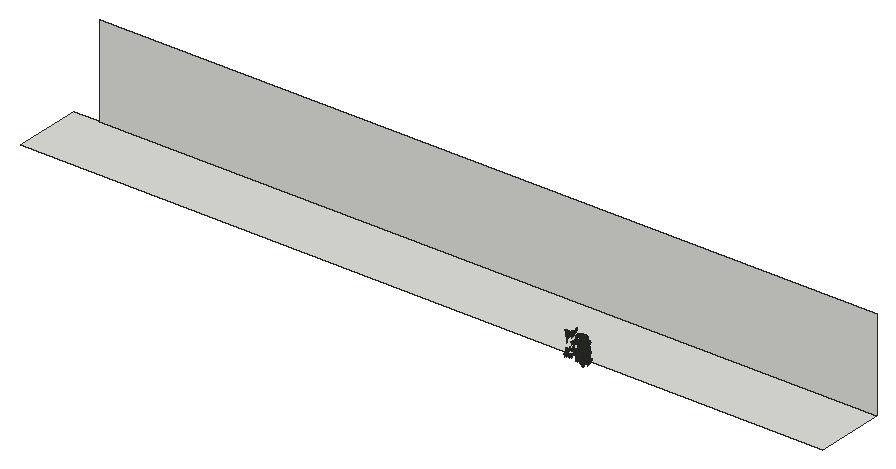
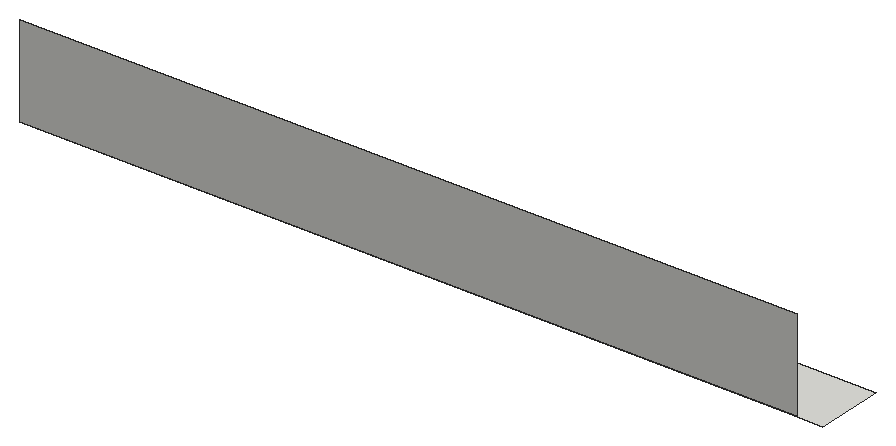
# SketchUp Ruby script. Lengths in inches.
U = 1.inch
M = Sketchup.active_model
def pt(a) = Geom::Point3d.new(a.map { |v| v * U })
def face(e, loops, mat)
  f = e.add_face(loops[0].map { |a| pt(a) })
  loops[1..].each { |l| e.add_face(l.map { |a| pt(a) }).erase! }
  f.material = f.back_material = mat if mat
  f
end
# faces: each face lists its corners as indices into pts; further lists are holes
def faces(e, pts, list, mat = nil) = list.each { |f| face(e, (f[0].is_a?(Array) ? f : [f]).map { |l| l.map { |i| pts[i] } }, mat) }
# xy, xz, yz: faces in a plane at the given z, y or x. An outline is a flat list of corners, or four numbers for a rectangle; further outlines are holes
def ring(l) = l.size == 4 ? [[l[0], l[1]], [l[2], l[1]], [l[2], l[3]], [l[0], l[3]]] : l.each_slice(2).to_a
def flat(e, list, mat, &to3) = list.each { |f| face(e, (f[0].is_a?(Array) ? f : [f]).map { |l| ring(l).map { |u, v| to3.(u, v) } }, mat) }
def xy(e, z, list, mat = nil) = flat(e, list, mat) { |x, y| [x, y, z] }
def xz(e, y, list, mat = nil) = flat(e, list, mat) { |x, z| [x, y, z] }
def yz(e, x, list, mat = nil) = flat(e, list, mat) { |y, z| [x, y, z] }
def lines(e, pts, list) = list.each { |a, b| e.add_line(pt(pts[a]), pt(pts[b])) }
# prism: a flat outline (further loops are holes) pulled along v
def prism(e, loops, v, mat = nil)
  f = face(e, loops, mat); d = Geom::Vector3d.new(v.map { |x| x * U })
  f.pushpull(f.normal.samedirection?(d) ? d.length : -d.length)
end
def box(e, o, s, mat = nil) = prism(e, [[o, [o[0] + s[0], o[1], o[2]], [o[0] + s[0], o[1] + s[1], o[2]], [o[0], o[1] + s[1], o[2]]]], [0, 0, s[2]], mat)
def at(x, y, z, deg = 0) = Geom::Transformation.translation(pt([x, y, z])) * Geom::Transformation.rotation(ORIGIN, Z_AXIS, deg.degrees)
def axes(o, x, y, z) = Geom::Transformation.new([*x, 0, *y, 0, *z, 0, *pt(o).to_a, 1])
def part(name) = M.definitions.add(name)
# library, detail: a bought-in or finely detailed component or shape, given as its bounding box
def library(name, o, s) = part(name).tap { |d| box(d.entities, o, s) }
def detail(e, o, s) = box(e.add_group.entities, o, s)
def put(e, d, t, mat = nil) = e.add_instance(d, t).tap { |i| i.material = mat if mat }
def group(e, t, mat = nil) = e.add_group.tap { |g| g.transformation = t; g.material = mat if mat }.entities
root = M.entities
M.materials.add("efeu2").color = [43, 57, 29]
c1 = part("ivyleaf_10")
p = [[0,0.5,-0.03],[-0.0625,2.02,-0.43],[-0.19,2.01,-0.46],[-0.54,1.05,-0.29],[-0.52,0.625,-0.18],[-0.83,0.76,-0.28],
  [-1.16,0.64,-0.33],[-1.15,0.33,-0.24],[-0.77,-0.39,0.02],[-0.3,-0.51,0.16],[0.04,-0.48,0.23],[-0.02,2.01,-0.4375],
  [-0.06,2.01,-0.43],[0.04,-0.49,0.23],[0.67,-0.49,0.14],[1.38,0.36,-0.2],[1.375,0.51,-0.24],[0.81,0.65,-0.19],
  [0.62,0.59,-0.15],[0.6,1.09,-0.28],[0.5,1.23,-0.31]]
faces(c1.entities,p,[[0,1,2,3,4,5,6,7,8,9,10],[11,12,0,13,14,15,16,17,18,19,20]],"efeu2")
xy(root,171.1,[[244.16,136.53,600.49,142.28,600,172.6875,260.85,167.21,243.67,166.9375]])
p = [[600,172.6875,212.04],[255.63,166.9375,212.04],[255.63,166.9375,171.1],[600,172.6875,171.1]]
faces(root,p,[[0,1,2,3]])
put(root,c1,axes([489.34,136.92,173.03],[-0.60098,-0.21353,-0.03623],[0.03346,0.01404,-0.63778],[0.21398,-0.6019,-0.00202]))
put(root,c1,axes([489.43,136.6,173.28],[0.58647,-0.26381,-0.03342],[-0.02854,0.01802,-0.64306],[0.26438,0.58715,0.00472]))
put(root,c1,axes([490.09,138.02,180.64],[0.42262,0.38706,-0.36071],[-0.30104,-0.20372,-0.57131],[-0.43509,0.51692,0.04493]))
put(root,c1,axes([490.55,136.09,175.51],[-0.59412,-0.11611,0.28646],[-0.27364,-0.09105,-0.60444],[0.14373,-0.65326,0.03333]))
put(root,c1,axes([490.71,136.64,182.22],[-0.56971,-0.26439,0.28808],[-0.2226,-0.19924,-0.62307],[0.32147,-0.60652,0.0791]))
put(root,c1,axes([490.89,135.48,183.34],[-0.63234,-0.11839,0.28705],[-0.27834,-0.07257,-0.64307],[0.13764,-0.69065,0.01836]))
put(root,c1,axes([490.71,135.68,180.78],[0.31183,-0.58954,-0.18764],[-0.09439,0.16234,-0.66689],[0.61144,0.32572,-0.00725]))
put(root,c1,axes([490.58,135.86,179.73],[0.43066,-0.5271,0.10645],[0.06697,-0.08274,-0.68066],[0.53355,0.43583,-0.00049]))
put(root,c1,axes([490.59,137.875,181.07],[0.07618,0.67726,0.04064],[-0.00515,0.04147,-0.68146],[-0.67846,0.07573,0.00973]))
put(root,c1,axes([490.84,135.45,182.15],[0.12255,-0.35746,0.58793],[-0.22289,0.54436,0.37743],[-0.65097,-0.25368,-0.01856]))
put(root,c1,axes([491.11,135.58,182.32],[-0.0211,-0.68119,-0.18478],[0.01976,0.18422,-0.68138],[0.70553,-0.02553,0.01355]))
put(root,c1,axes([491.64,135.9,176.41],[0.32546,-0.42345,-0.42045],[-0.09516,0.43596,-0.51273],[0.58909,0.30437,0.14946]))
put(root,c1,axes([491.76,137.48,182.52],[-0.22643,-0.65307,0.02889],[-0.00889,-0.02749,-0.69121],[0.65365,-0.22661,0.0006]))
put(root,c1,axes([491.77,137.86,178.3],[-0.12532,-0.5727,0.31845],[0.05902,-0.33277,-0.57522],[0.65262,-0.07988,0.11318]))
put(root,c1,axes([491.84,136.24,173.86],[-0.00285,-0.61174,0.26083],[0.02269,-0.26077,-0.61135],[0.66464,0.00628,0.02199]))
put(root,c1,axes([491.94,138.29,174.82],[-0.05674,-0.6367,0.11101],[0.00067,-0.1115,-0.63914],[0.6463,-0.05578,0.01041]))
put(root,c1,axes([492.33,136.56,173.53],[0.28308,-0.51776,-0.30381],[-0.13114,0.27445,-0.58991],[0.58581,0.31164,0.01475]))
put(root,c1,axes([492.51,137.45,182.44],[-0.20031,-0.64966,0.13016],[0.01179,-0.13945,-0.67789],[0.66247,-0.19395,0.05142]))
put(root,c1,axes([492.42,138.36,173.77],[0.11732,-0.58138,-0.2462],[0.08014,0.26211,-0.58075],[0.62626,0.07537,0.12044]))
put(root,c1,axes([492.72,137.77,179.57],[0.24028,-0.62845,-0.07217],[-0.00763,0.07432,-0.67255],[0.63254,0.23963,0.0193]))
put(root,c1,axes([492.92,135.86,176.87],[0.08003,-0.47649,-0.4878],[0.00128,0.49125,-0.47965],[0.6819,0.05499,0.05815]))
put(root,c1,axes([493.3125,137.41,183.74],[0.27388,-0.55892,-0.32588],[-0.07106,0.32574,-0.61842],[0.64307,0.27404,0.07045]))
put(root,c1,axes([493.3125,137.84,179.09],[0.09889,-0.63502,-0.20371],[-0.03774,0.20028,-0.64264],[0.66583,0.10567,-0.00617]))
put(root,c1,axes([493.85,137.6,181.86],[-0.09441,-0.68576,-0.01445],[0.00171,0.01435,-0.69223],[0.68591,-0.09443,-0.00026]))
put(root,c1,axes([494.01,138.49,172.42],[-0.2121,-0.59835,-0.04185],[0.01001,0.04086,-0.63482],[0.59973,-0.2123,-0.0042]))
put(root,c1,axes([494.11,138.23,175.14],[-0.04112,-0.64651,0.07347],[-0.00293,-0.07344,-0.64781],[0.65066,-0.04119,0.00173]))
put(root,c1,axes([494.27,136.76,172.6],[0.50384,-0.21043,-0.3824],[-0.26182,0.32157,-0.52193],[0.34923,0.54468,0.1604]))
put(root,c1,axes([494.24,135.48,180.08],[-0.01693,-0.68539,0.18089],[0.04753,-0.18163,-0.68375],[0.70726,-0.0042,0.05028]))
put(root,c1,axes([494.32,137.8,179.27],[0.09713,-0.65896,-0.1229],[0.0085,0.12538,-0.66557],[0.67027,0.0939,0.02625]))
put(root,c1,axes([494.56,137.95,173.88],[-0.61745,-0.07231,0.17501],[-0.17585,-0.00247,-0.62142],[0.07024,-0.64176,-0.01733]))
put(root,c1,axes([494.47,137.84,174.24],[0.46469,-0.12531,0.43496],[0.42427,-0.09668,-0.48112],[0.15777,0.62911,0.0127]))
put(root,c1,axes([494.94,138.15,175.62],[-0.26579,-0.5574,0.22476],[-0.00438,-0.24396,-0.61018],[0.60099,-0.24829,0.09496]))
put(root,c1,axes([494.8,137.88,174.74],[-0.57989,0.06979,-0.28827],[0.28028,-0.07811,-0.58274],[-0.09701,-0.64286,0.03951]))
put(root,c1,axes([494.74,137.52,174.21],[0.63442,0.13863,0.1945],[0.18349,0.07053,-0.64877],[-0.15291,0.65981,0.02849]))
put(root,c1,axes([495.33,137.22,176.72],[0.47629,-0.0279,-0.50428],[-0.50255,0.04266,-0.47702],[0.05016,0.69233,0.00907]))
put(root,c1,axes([495.28,137.48,172.41],[0.33532,-0.53591,-0.09551],[-0.06548,0.07165,-0.63193],[0.5404,0.34122,-0.01731]))
put(root,c1,axes([495.41,137.43,172.87],[0.43742,-0.27794,-0.37958],[-0.25033,0.30133,-0.50912],[0.39833,0.49459,0.09687]))
put(root,c1,axes([495.53,137.66,173.3],[-0.23084,0.51009,0.32121],[-0.15983,0.27986,-0.55928],[-0.58122,-0.27955,0.02622]))
put(root,c1,axes([495.59,137.84,178.86],[-0.03666,0.6764,0.00446],[-0.00017,0.00445,-0.67739],[-0.67641,-0.03666,-0.00007]))
put(root,c1,axes([495.7,135.62,179.77],[0.1972,-0.48675,-0.48127],[0.02925,0.50638,-0.50016],[0.68388,0.1187,0.16017]))
put(root,c1,axes([495.65,137.25,182.1],[0.05159,-0.51268,0.47251],[0.17952,-0.44805,-0.50575],[0.6737,0.15865,0.09858]))
put(root,c1,axes([495.9,137.51,176.07],[-0.37959,-0.50761,0.18659],[-0.0422,-0.19947,-0.6285],[0.53917,-0.37298,0.08217]))
put(root,c1,axes([495.93,136.68,181.83],[0.27902,-0.56461,-0.35008],[-0.15993,0.31145,-0.62977],[0.6448,0.32157,-0.00471]))
put(root,c1,axes([495.91,138.03,175.22],[-0.5594,-0.33047,0.09999],[-0.01373,-0.16892,-0.63514],[0.34499,-0.54257,0.13684]))
put(root,c1,axes([495.75,137.53,179.64],[0.43201,-0.52624,0.02536],[0.0041,0.03615,0.68035],[-0.52684,-0.43124,0.02609]))
put(root,c1,axes([496.0625,137.16,175.76],[-0.53956,-0.38209,-0.00867],[0.00845,0.00307,-0.66115],[0.3821,-0.53962,0.00238]))
put(root,c1,axes([496.14,137.59,180.86],[-0.26919,-0.63261,0.04342],[0.04286,-0.06521,-0.68443],[0.63265,-0.26475,0.06485]))
put(root,c1,axes([496.23,137.15,175.59],[0.30439,0.44445,-0.38843],[-0.29247,-0.26605,-0.53361],[-0.51271,0.41563,0.07379]))
put(root,c1,axes([496.09,136.69,174.4375],[-0.51645,-0.35862,-0.18748],[0.17519,0.07588,-0.62772],[0.36479,-0.54416,0.03603]))
put(root,c1,axes([496.16,137.34,180.05],[-0.12572,0.56866,0.35734],[-0.09397,0.34508,-0.58221],[-0.66501,-0.15627,0.01471]))
put(root,c1,axes([496.25,137.57,181.35],[-0.35976,-0.58708,0.07461],[0.0274,-0.10375,-0.68421],[0.59117,-0.35246,0.07711]))
put(root,c1,axes([496.49,136.64,176.6],[-0.64085,0.08234,0.16507],[-0.17268,-0.0579,-0.64152],[-0.06488,-0.65923,0.07696]))
put(root,c1,axes([496.25,135.99,178.7],[-0.10275,-0.42425,-0.55999],[0.17824,0.53169,-0.43552],[0.67956,-0.2036,0.02956]))
put(root,c1,axes([496.83,136.26,172.86],[0.04499,-0.04104,-0.7294],[-0.66354,0.30345,-0.058],[0.30565,0.6648,-0.01855]))
put(root,c1,axes([496.25,136.34,173.23],[0.04748,0.2806,0.64845],[0.00029,0.6499,-0.28125],[-0.70655,0.01912,0.04346]))
put(root,c1,axes([496.16,137.61,180.9],[0.52095,0.43636,0.1171],[0.09012,0.07478,-0.67956],[-0.44272,0.52869,-0.00054]))
put(root,c1,axes([496.33,137.5625,181.76],[0.53937,0.42733,-0.09746],[-0.13135,0.01015,-0.68241],[-0.41816,0.54801,0.08864]))
put(root,c1,axes([496.45,136.01,178.68],[0.4186,-0.54431,-0.18352],[-0.06381,0.1816,-0.6842],[0.57086,0.41944,0.05808]))
put(root,c1,axes([496.48,136.79,181.5],[-0.3137,-0.63775,-0.11816],[0.05901,0.10265,-0.71069],[0.64592,-0.31911,0.00754]))
put(root,c1,axes([496.38,138.23,173.49],[-0.07086,0.63887,-0.1144],[0.00011,-0.11507,-0.64267],[-0.64904,-0.06977,0.01238]))
put(root,c1,axes([496.67,138.22,172.46],[-0.51858,-0.29802,0.24077],[-0.08922,-0.30011,-0.56363],[0.37259,-0.48665,0.20014]))
put(root,c1,axes([496.4,137.54,182.02],[-0.25128,-0.34217,-0.55231],[0.33937,0.43584,-0.42442],[0.55403,-0.42217,0.00948]))
put(root,c1,axes([496.81,138.13,174.65],[-0.33876,-0.45424,0.33849],[-0.17119,-0.29387,-0.56569],[0.54001,-0.37812,0.03301]))
put(root,c1,axes([496.59,137.05,177.89],[-0.35333,-0.55847,-0.13766],[0.13318,0.07773,-0.65719],[0.55955,-0.37115,0.06949]))
put(root,c1,axes([496.63,137.86,175.74],[0.07001,-0.56152,-0.34486],[0.08579,0.35162,-0.55511],[0.65336,0.014,0.10984]))
put(root,c1,axes([496.56,138.18,173.9375],[0.02236,0.65463,-0.0365],[-0.00132,-0.03648,-0.65501],[-0.65564,0.0224,0.00007]))
put(root,c1,axes([496.76,135.76,180.41],[0.24437,-0.32979,-0.5934],[-0.01348,0.62819,-0.35468],[0.67875,0.13121,0.20659]))
put(root,c1,axes([496.57,136.59,183.34],[-0.0171,-0.6732,0.28474],[0.36584,-0.25446,-0.57963],[0.6328,0.12892,0.3428]))
put(root,c1,axes([496.78,138.09,174.73],[0.00548,-0.48929,0.44481],[0.09398,-0.43973,-0.48486],[0.65454,0.06724,0.0659]))
put(root,c1,axes([496.875,137.73,178.4],[0.34431,-0.54496,-0.20928],[-0.05274,0.21293,-0.64125],[0.58137,0.34206,0.06577]))
put(root,c1,axes([496.91,138.15,174.34],[0.11847,-0.64019,-0.09152],[-0.00044,0.09296,-0.65086],[0.6467,0.11734,0.01632]))
put(root,c1,axes([496.87,137.07,178.74],[-0.20858,-0.59069,-0.26106],[0.11065,0.23759,-0.626],[0.63626,-0.23496,0.02328]))
put(root,c1,axes([496.95,137.42,182.1],[0.01766,-0.69736,0.01255],[-0.00193,-0.0126,-0.69758],[0.69747,0.01762,-0.00225]))
put(root,c1,axes([496.42,138.25,173.58],[0.22849,0.10897,0.60259],[0.54939,0.24761,-0.25309],[-0.27048,0.59499,-0.00503]))
put(root,c1,axes([496.95,137.12,180.78],[-0.71446,0.1047,-0.07512],[0.07393,-0.01356,-0.72209],[-0.10554,-0.71827,0.00268]))
put(root,c1,axes([497.16,136.02,177.83],[-0.63943,-0.18104,0.13771],[-0.13193,-0.03952,-0.66456],[0.18529,-0.65289,0.00204]))
put(root,c1,axes([496.9375,136.93,179.08],[-0.61512,0.28049,-0.09416],[0.08418,-0.04234,-0.67604],[-0.28364,-0.62085,0.00356]))
put(root,c1,axes([497.43,137.01,180.23],[0.40014,-0.07642,-0.55362],[-0.54216,0.11214,-0.40734],[0.13561,0.67381,0.005]))
put(root,c1,axes([497.29,137.55,179.35],[-0.04139,-0.67113,0.12702],[-0.0146,-0.12635,-0.67237],[0.68289,-0.04338,-0.00668]))
put(root,c1,axes([497.28,137.92,176.48],[-0.19927,-0.6345,-0.1009],[0.01326,0.10155,-0.66482],[0.64234,-0.19893,-0.01758]))
put(root,c1,axes([497.32,138.02,175.6],[-0.12881,-0.65142,-0.05506],[0.00536,0.05506,-0.66401],[0.65372,-0.12881,-0.00541]))
put(root,c1,axes([497.32,137.36,179.94],[-0.68579,-0.04189,-0.0047],[0.00469,0.00025,-0.68707],[0.04189,-0.68581,0.00004]))
put(root,c1,axes([497.67,137.61,172.37],[0.40607,-0.02268,-0.50401],[-0.44402,0.29111,-0.37084],[0.23954,0.57807,0.16698]))
put(root,c1,axes([497.5,136.3125,175.02],[0.27515,-0.46226,-0.39053],[-0.09285,0.39168,-0.52903],[0.59798,0.27352,0.09755]))
put(root,c1,axes([497.4375,137.92,176.72],[0.06427,0.43176,0.51307],[-0.09181,0.51623,-0.42292],[-0.66425,-0.02957,0.1081]))
put(root,c1,axes([497.14,135.96,171.75],[-0.51324,0.05015,0.53885],[0.53259,-0.08498,0.51519],[0.09603,0.73929,0.02267]))
put(root,c1,axes([497.51,137.91,173.4],[0.27999,-0.61772,0.01758],[0.00744,-0.01592,-0.67821],[0.61793,0.28008,0.0002]))
put(root,c1,axes([497.69,136.86,180.13],[-0.17132,-0.67874,-0.19466],[0.09507,0.17631,-0.69843],[0.69967,-0.19015,0.04724]))
put(root,c1,axes([497.86,137.74,178.33],[0.44391,0.35841,-0.37874],[-0.30817,-0.22092,-0.57025],[-0.42064,0.54009,0.01808]))
put(root,c1,axes([497.55,137,180.41],[-0.3059,-0.44364,-0.48768],[0.36468,0.33402,-0.5326],[0.54924,-0.46887,0.08202]))
put(root,c1,axes([497.86,137.72,178.45],[-0.04616,-0.67224,-0.12382],[0.01068,0.12338,-0.67382],[0.68346,-0.04733,0.00217]))
put(root,c1,axes([497.78,136.57,180.1],[-0.67089,-0.12742,-0.14668],[0.14512,0.022,-0.68286],[0.1292,-0.68638,0.00534]))
put(root,c1,axes([497.76,136.45,178.4],[0.68176,-0.20634,0.0203],[0.02042,-0.00261,-0.71229],[0.20632,0.68206,0.00342]))
put(root,c1,axes([497.95,138.32,172.05],[-0.07008,-0.64013,0.02762],[0.00488,-0.02831,-0.64391],[0.64071,-0.0698,0.00792]))
put(root,c1,axes([498.16,136.65,182.625],[-0.3232,-0.3307,0.57903],[-0.22009,-0.5545,-0.43954],[0.62945,-0.36369,0.14363]))
put(root,c1,axes([497.47,137.62,174.12],[0.35436,-0.19668,0.54592],[0.55796,-0.06016,-0.38385],[0.15934,0.64806,0.13004]))
put(root,c1,axes([498.06,138.22,172.66],[-0.12087,-0.60941,0.17977],[-0.04457,-0.17441,-0.62121],[0.63381,-0.12849,-0.0094]))
put(root,c1,axes([498.09,137.75,177.59],[-0.36917,-0.566,0.05797],[-0.02731,-0.05139,-0.67573],[0.5683,-0.37015,0.00518]))
put(root,c1,axes([497.91,135.4375,182.58],[0.25462,0.69147,-0.15025],[-0.05257,-0.14076,-0.73686],[-0.70565,0.25999,0.00068]))
put(root,c1,axes([498,137.84,177.4375],[0.41651,-0.51225,-0.15366],[0.00626,0.19942,-0.64783],[0.53476,0.39664,0.12727]))
put(root,c1,axes([498.07,137.51,175.75],[0.67979,-0.07946,-0.10379],[-0.10136,0.02668,-0.68427],[0.08255,0.68715,0.01456]))
put(root,c1,axes([497.9,137.11,174.03],[0.0121,0.03073,0.69844],[0.16932,0.67762,-0.03275],[-0.6783,0.16969,0.00429]))
put(root,c1,axes([497.92,137.1,174.63],[0.21011,-0.42483,0.51244],[0.30878,-0.41384,-0.4697],[0.58969,0.36807,0.06336]))
put(root,c1,axes([498.23,138.18,174.6875],[-0.05966,-0.65426,-0.02118],[-0.00921,0.0221,-0.65688],[0.65454,-0.05932,-0.01117]))
put(root,c1,axes([498.21,137.8,177.81],[0.26954,-0.59828,-0.18198],[-0.00391,0.19655,-0.65196],[0.62533,0.2591,0.07437]))
put(root,c1,axes([498.15,137.63,179.29],[-0.08073,0.68418,-0.04311],[0.0019,-0.04318,-0.68892],[-0.68553,-0.08069,0.00317]))
put(root,c1,axes([498.31,137.71,178.96],[0.30486,-0.55116,-0.27285],[0.00015,0.30461,-0.61513],[0.615,0.27314,0.13541]))
put(root,c1,axes([498.38,137.75,176.54],[-0.28388,-0.59707,0.11599],[0.00899,-0.1321,-0.65803],[0.60816,-0.27674,0.06387]))
put(root,c1,axes([498.45,138.14,172.16],[-0.28564,-0.52681,0.236],[-0.02043,-0.25391,-0.59154],[0.57689,-0.26983,0.0959]))
put(root,c1,axes([498.43,137.75,178.11],[-0.20208,-0.64927,-0.03225],[0.01409,0.02939,-0.67998],[0.64992,-0.20252,0.00472]))
put(root,c1,axes([498.43,136.75,176.22],[0.08907,-0.69335,0.14255],[0.03334,-0.1394,-0.69889],[0.70707,0.09391,0.01499]))
put(root,c1,axes([498.52,138.34,173.07],[-0.0486,-0.63599,0.10402],[-0.0159,-0.1031,-0.6378],[0.64425,-0.05052,-0.00789]))
put(root,c1,axes([498.4,135.24,182.64],[0.37557,0.59901,-0.28593],[0.13589,0.25217,0.70679],[0.64969,-0.39902,0.01745]))
put(root,c1,axes([498.62,136.56,177.7],[-0.16978,-0.68666,0.12516],[-0.03284,-0.12081,-0.70733],[0.6972,-0.1729,-0.00283]))
put(root,c1,axes([498.625,137.53,180.01],[-0.37473,-0.5705,0.12323],[-0.00321,-0.14442,-0.67838],[0.58365,-0.36708,0.07539]))
put(root,c1,axes([498.75,136.45,177.19],[-0.04306,-0.17047,0.69788],[-0.15766,-0.67984,-0.17579],[0.70088,-0.16341,0.00333]))
put(root,c1,axes([498.69,137.85,176.38],[-0.42038,-0.50018,0.15074],[-0.03421,-0.16671,-0.64858],[0.52128,-0.41431,0.07899]))
put(root,c1,axes([498.59,138,175.04],[0.17793,-0.574,-0.2759],[0.05229,0.29867,-0.58764],[0.63472,0.1363,0.12575]))
put(root,c1,axes([498.77,136.11,183.38],[0.62332,0.08857,-0.34913],[-0.3414,-0.07721,-0.62909],[-0.11484,0.71025,-0.02485]))
put(root,c1,axes([498.56,137.41,174.98],[-0.14273,0.59603,-0.26917],[0.00285,-0.27494,-0.61031],[-0.65398,-0.13128,0.05609]))
put(root,c1,axes([498.78,137.28,177.85],[-0.26962,-0.53898,0.30992],[-0.06533,-0.31138,-0.59835],[0.61829,-0.26794,0.07193]))
put(root,c1,axes([498.85,138.21,173.47],[-0.4986,-0.37717,0.18792],[-0.06046,-0.22408,-0.61017],[0.41703,-0.48343,0.13621]))
put(root,c1,axes([498.67,137.52,180.62],[-0.47063,-0.51286,-0.07817],[0.19531,-0.07739,-0.6682],[0.48061,-0.47076,0.195]))
